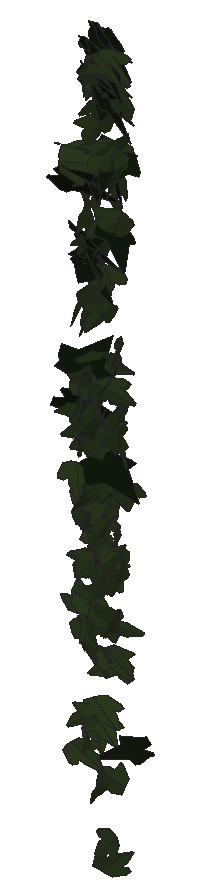
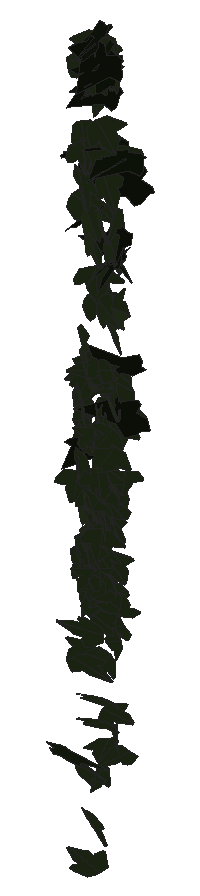
# SketchUp Ruby script. Lengths in inches.
U = 1.inch
M = Sketchup.active_model
def pt(a) = Geom::Point3d.new(a.map { |v| v * U })
def face(e, loops, mat)
  f = e.add_face(loops[0].map { |a| pt(a) })
  loops[1..].each { |l| e.add_face(l.map { |a| pt(a) }).erase! }
  f.material = f.back_material = mat if mat
  f
end
# faces: each face lists its corners as indices into pts; further lists are holes
def faces(e, pts, list, mat = nil) = list.each { |f| face(e, (f[0].is_a?(Array) ? f : [f]).map { |l| l.map { |i| pts[i] } }, mat) }
# xy, xz, yz: faces in a plane at the given z, y or x. An outline is a flat list of corners, or four numbers for a rectangle; further outlines are holes
def ring(l) = l.size == 4 ? [[l[0], l[1]], [l[2], l[1]], [l[2], l[3]], [l[0], l[3]]] : l.each_slice(2).to_a
def flat(e, list, mat, &to3) = list.each { |f| face(e, (f[0].is_a?(Array) ? f : [f]).map { |l| ring(l).map { |u, v| to3.(u, v) } }, mat) }
def xy(e, z, list, mat = nil) = flat(e, list, mat) { |x, y| [x, y, z] }
def xz(e, y, list, mat = nil) = flat(e, list, mat) { |x, z| [x, y, z] }
def yz(e, x, list, mat = nil) = flat(e, list, mat) { |y, z| [x, y, z] }
def lines(e, pts, list) = list.each { |a, b| e.add_line(pt(pts[a]), pt(pts[b])) }
# prism: a flat outline (further loops are holes) pulled along v
def prism(e, loops, v, mat = nil)
  f = face(e, loops, mat); d = Geom::Vector3d.new(v.map { |x| x * U })
  f.pushpull(f.normal.samedirection?(d) ? d.length : -d.length)
end
def box(e, o, s, mat = nil) = prism(e, [[o, [o[0] + s[0], o[1], o[2]], [o[0] + s[0], o[1] + s[1], o[2]], [o[0], o[1] + s[1], o[2]]]], [0, 0, s[2]], mat)
def at(x, y, z, deg = 0) = Geom::Transformation.translation(pt([x, y, z])) * Geom::Transformation.rotation(ORIGIN, Z_AXIS, deg.degrees)
def axes(o, x, y, z) = Geom::Transformation.new([*x, 0, *y, 0, *z, 0, *pt(o).to_a, 1])
def part(name) = M.definitions.add(name)
# library, detail: a bought-in or finely detailed component or shape, given as its bounding box
def library(name, o, s) = part(name).tap { |d| box(d.entities, o, s) }
def detail(e, o, s) = box(e.add_group.entities, o, s)
def put(e, d, t, mat = nil) = e.add_instance(d, t).tap { |i| i.material = mat if mat }
def group(e, t, mat = nil) = e.add_group.tap { |g| g.transformation = t; g.material = mat if mat }.entities
root = M.entities
M.materials.add("1026 AP 7946 SUNNY SIDE UP").color = [254, 231, 186]
M.materials.add("efeu1").color = [18, 25, 13]
M.materials.add("efeu2").color = [43, 57, 29]
c1 = part("ivyleaf_10")
p = [[0,0.5,-0.03],[-0.0625,2.02,-0.43],[-0.19,2.01,-0.46],[-0.54,1.05,-0.29],[-0.52,0.625,-0.18],[-0.83,0.76,-0.28],
  [-1.16,0.64,-0.33],[-1.15,0.33,-0.24],[-0.77,-0.39,0.02],[-0.3,-0.51,0.16],[0.04,-0.48,0.23],[-0.02,2.01,-0.4375],
  [-0.06,2.01,-0.43],[0.04,-0.49,0.23],[0.67,-0.49,0.14],[1.38,0.36,-0.2],[1.375,0.51,-0.24],[0.81,0.65,-0.19],
  [0.62,0.59,-0.15],[0.6,1.09,-0.28],[0.5,1.23,-0.31]]
faces(c1.entities,p,[[0,1,2,3,4,5,6,7,8,9,10],[11,12,0,13,14,15,16,17,18,19,20]],"efeu2")
c2 = part("ivyleaf_9")
p = [[1.54,2.16,1.25],[1.36,2.04,1.19],[-0.21,0.99,0.68],[-0.71,1.11,0.82],[-0.85,0.86,0.67],[-0.8,0.17,0.21],
  [-0.9,-0.01,0.1],[-0.67,-0.16,-0.02],[-0.08,-0.08,-0.05],[-0.03,-0.6,-0.4],[0.65,-0.88,-0.66],[0.83,-0.6,-0.49],
  [1.29,-0.42,-0.43],[1.8125,-0.07,-0.26],[1.21,0.44,0.15]]
faces(c2.entities,p,[[0,1,2,3,4,5,6,7,8,9,10,11,12,13,14]],"efeu1")
put(root,c1,axes([100.83,212.89,262.52],[0.13665,-0.19544,0.01189],[-0.00323,-0.01554,-0.22635],[0.33256,0.08016,-0.00708]),"1026 AP 7946 SUNNY SIDE UP")
put(root,c1,axes([100.85,212.84,264.03],[-0.01043,-0.23526,0.01809],[-0.0003,-0.0189,-0.24257],[0.37111,-0.00663,0.00031]),"1026 AP 7946 SUNNY SIDE UP")
put(root,c1,axes([100.76,212.64,259.7],[0.25132,0.14631,-0.00572],[0.00915,-0.01575,-0.22248],[-0.2485,0.14739,-0.01398]),"1026 AP 7946 SUNNY SIDE UP")
put(root,c2,axes([100.73,212.62,265.69],[0.37967,0.09039,0.01328],[-0.0411,0.0877,-0.23827],[-0.14905,0.20606,0.09953]),"1026 AP 7946 SUNNY SIDE UP")
put(root,c1,axes([100.84,212.66,257.16],[0.28828,0.09088,0.01076],[-0.02972,0.01592,0.2096],[0.14064,-0.18291,0.02224]),"1026 AP 7946 SUNNY SIDE UP")
put(root,c1,axes([100.77,212.8,262.84],[0.07996,-0.1274,0.21096],[0.12187,-0.19033,-0.14243],[0.36013,0.09269,0.00136]),"1026 AP 7946 SUNNY SIDE UP")
put(root,c1,axes([100.91,212.78,258.08],[-0.13223,-0.16283,0.09855],[-0.02891,-0.09816,-0.18755],[0.29628,-0.08225,0.02568]),"1026 AP 7946 SUNNY SIDE UP")
put(root,c1,axes([100.79,213.01,260.64],[-0.28985,0.02637,-0.0702],[0.10092,-0.04074,-0.18288],[-0.06588,-0.17844,0.02871]),"1026 AP 7946 SUNNY SIDE UP")
put(root,c2,axes([100.5625,212.65,260.9375],[0.09228,0.04957,-0.24052],[0.24625,0.17382,0.0795],[0.28379,-0.16695,0.00923]),"1026 AP 7946 SUNNY SIDE UP")
put(root,c1,axes([100.89,212.6,260.89],[-0.27426,-0.1545,-0.00761],[0.02677,-0.00944,-0.23935],[0.24167,-0.17429,0.01788]),"1026 AP 7946 SUNNY SIDE UP")
put(root,c1,axes([100.89,212.53,261.15],[0.09027,-0.1714,-0.14386],[-0.00129,0.14312,-0.18177],[0.34667,0.04517,0.03678]),"1026 AP 7946 SUNNY SIDE UP")
put(root,c1,axes([100.76,212.92,258.92],[0.25824,-0.10235,0.08625],[0.12248,-0.03414,-0.19922],[0.16873,0.18143,0.01261]),"1026 AP 7946 SUNNY SIDE UP")
put(root,c1,axes([100.76,213.21,264.56],[0.16686,-0.11265,0.14808],[0.14553,-0.11057,-0.16148],[0.26777,0.13029,-0.00452]),"1026 AP 7946 SUNNY SIDE UP")
put(root,c1,axes([100.63,212.77,261.42],[-0.02711,-0.01639,-0.22131],[0.29318,-0.11543,-0.00611],[-0.19419,-0.17198,0.02168]),"1026 AP 7946 SUNNY SIDE UP")
put(root,c1,axes([100.82,212.64,260.21],[-0.15831,0.14303,0.13806],[0.14235,-0.09653,0.18083],[0.29194,0.12462,-0.01331]),"1026 AP 7946 SUNNY SIDE UP")
put(root,c2,axes([100.6,212.48,265.16],[0.35763,0.03996,0.12969],[0.20161,-0.00852,-0.23633],[-0.04841,0.25971,-0.02615]),"1026 AP 7946 SUNNY SIDE UP")
put(root,c1,axes([100.91,212.77,258.98],[0.11899,-0.1979,-0.00095],[-0.00676,-0.00186,-0.21824],[0.31111,0.07565,-0.00438]),"1026 AP 7946 SUNNY SIDE UP")
put(root,c1,axes([100.86,212.71,264.49],[0.0494,-0.19948,-0.13684],[0.07459,0.13539,-0.19882],[0.36838,-0.00066,0.05861]),"1026 AP 7946 SUNNY SIDE UP")
put(root,c1,axes([100.89,213.03,257.93],[-0.27474,0.0567,-0.04591],[0.02238,-0.08242,-0.1682],[-0.11937,-0.14596,0.07414]),"1026 AP 7946 SUNNY SIDE UP")
put(root,c1,axes([100.78,213,257.7],[-0.2358,0.00664,-0.1185],[0.17399,-0.06035,-0.14231],[-0.07221,-0.1671,0.04405]),"1026 AP 7946 SUNNY SIDE UP")
put(root,c2,axes([100.87,212.69,263.85],[0.26545,-0.09188,-0.16491],[-0.22705,0.06825,-0.19747],[0.17963,0.22204,-0.0059]),"1026 AP 7946 SUNNY SIDE UP")
put(root,c1,axes([100.84,212.57,261.37],[0.04187,0.00239,0.24061],[0.00754,0.235,-0.00167],[-0.36717,0.0051,0.0274]),"1026 AP 7946 SUNNY SIDE UP")
put(root,c1,axes([100.82,212.93,257.8],[-0.17724,0.07081,-0.14009],[0.10843,-0.12422,-0.12737],[-0.22964,-0.1133,0.04799]),"1026 AP 7946 SUNNY SIDE UP")
put(root,c1,axes([100.93,212.48,259.08],[0.05187,-0.01626,0.23813],[-0.07855,0.22759,0.02516],[-0.35594,-0.0526,0.02915]),"1026 AP 7946 SUNNY SIDE UP")
put(root,c1,axes([101.02,212.6875,255.23],[-0.1167,-0.06502,0.16342],[-0.08392,-0.15062,-0.09411],[0.27025,-0.07484,0.04135]),"1026 AP 7946 SUNNY SIDE UP")
put(root,c1,axes([100.94,212.7,261.01],[0.10666,-0.21059,0.04081],[0.00753,-0.04131,-0.22802],[0.33721,0.06753,-0.00782]),"1026 AP 7946 SUNNY SIDE UP")
put(root,c1,axes([100.97,213.04,257.91],[-0.0692,-0.10126,0.14748],[-0.00023,-0.14291,-0.11343],[0.29204,-0.02411,0.03486]),"1026 AP 7946 SUNNY SIDE UP")
put(root,c1,axes([100.98,212.82,265.14],[-0.0718,-0.23668,0.02762],[-0.00268,-0.02834,-0.24846],[0.37478,-0.04555,0.00351]),"1026 AP 7946 SUNNY SIDE UP")
put(root,c1,axes([101.01,212.77,258.1],[-0.18106,-0.13037,0.1157],[-0.04366,-0.12014,-0.17256],[0.26779,-0.10773,0.05009]),"1026 AP 7946 SUNNY SIDE UP")
put(root,c1,axes([100.96,212.98,258.65],[-0.26566,-0.11815,-0.01533],[0.03451,-0.00668,-0.21162],[0.1839,-0.16942,0.01756]),"1026 AP 7946 SUNNY SIDE UP")
put(root,c1,axes([100.98,212.87,262.85],[0.00658,-0.2045,0.11564],[0.0091,-0.1133,-0.21135],[0.36757,0.00646,0.00316]),"1026 AP 7946 SUNNY SIDE UP")
put(root,c1,axes([100.78,212.62,254.52],[0.15606,0.11813,0.14604],[0.16222,0.09701,-0.15788],[-0.23959,0.14264,-0.01178]),"1026 AP 7946 SUNNY SIDE UP")
put(root,c1,axes([101.07,212.61,261.21],[-0.12313,0.15192,-0.16471],[-0.09578,0.14912,0.17663],[0.33434,0.09867,-0.01006]),"1026 AP 7946 SUNNY SIDE UP")
put(root,c1,axes([100.98,212.77,258.98],[-0.03758,-0.19625,0.06368],[0.01359,-0.06425,-0.20341],[0.32377,-0.02008,0.01593]),"1026 AP 7946 SUNNY SIDE UP")
put(root,c2,axes([100.85,212.625,261.58],[-0.18274,-0.00375,0.22652],[0.33447,0.06129,0.11724],[-0.08789,0.24105,-0.02479]),"1026 AP 7946 SUNNY SIDE UP")
put(root,c1,axes([100.9,212.83,260.15],[-0.31442,-0.05777,-0.07811],[0.12679,-0.00996,-0.21224],[0.07917,-0.2135,0.02969]),"1026 AP 7946 SUNNY SIDE UP")
put(root,c1,axes([100.95,212.68,267.12],[-0.27533,0.18064,-0.02232],[0.00585,-0.02792,-0.25877],[-0.28622,-0.17434,0.01618]),"1026 AP 7946 SUNNY SIDE UP")
put(root,c1,axes([101.03,212.9,266.17],[-0.1391,-0.21122,0.09816],[-0.01901,-0.09892,-0.23509],[0.36464,-0.08573,0.02519]),"1026 AP 7946 SUNNY SIDE UP")
put(root,c1,axes([100.9,212.94,254.83],[0.12092,0.19268,0.01725],[0.01968,0.01185,-0.21353],[-0.30334,0.07758,-0.00698]),"1026 AP 7946 SUNNY SIDE UP")
put(root,c1,axes([100.98,212.75,258.96],[-0.01835,-0.18616,-0.09728],[0.02667,0.09236,-0.19134],[0.32638,-0.01801,0.01017]),"1026 AP 7946 SUNNY SIDE UP")
put(root,c1,axes([100.98,212.5625,261.33],[0.01684,-0.02935,0.23079],[-0.0714,0.21959,0.03313],[-0.34828,-0.04644,0.00437]),"1026 AP 7946 SUNNY SIDE UP")
put(root,c1,axes([101.01,212.69,259.7],[0.10256,-0.21321,0.01528],[0.00009,-0.01676,-0.22974],[0.3362,0.06504,-0.0046]),"1026 AP 7946 SUNNY SIDE UP")
put(root,c2,axes([101.19,212.7,263.99],[-0.21293,0.19926,0.01856],[-0.02391,0.01007,-0.24803],[-0.31353,-0.13609,0.00632]),"1026 AP 7946 SUNNY SIDE UP")
put(root,c1,axes([100.78,212.81,259.21],[0.23154,0.04263,0.14785],[0.2289,0.02869,-0.15227],[-0.0858,0.19158,-0.00723]),"1026 AP 7946 SUNNY SIDE UP")
put(root,c1,axes([101.05,212.87,261.78],[-0.14826,-0.1957,0.06223],[-0.01221,-0.06425,-0.22321],[0.32234,-0.09245,0.02017]),"1026 AP 7946 SUNNY SIDE UP")
put(root,c1,axes([101,212.6,260.53],[-0.29341,-0.13473,-0.04142],[0.07203,0.00358,-0.23584],[0.20867,-0.19069,0.02317]),"1026 AP 7946 SUNNY SIDE UP")
put(root,c2,axes([100.9,212.89,265.42],[-0.01736,-0.24334,0.02718],[-0.00489,-0.02765,-0.2511],[0.38509,-0.01132,-0.00196]),"1026 AP 7946 SUNNY SIDE UP")
put(root,c1,axes([100.85,213.16,259.39],[0.24045,-0.01826,0.11366],[0.17273,-0.03608,-0.15215],[0.06126,0.17345,-0.01713]),"1026 AP 7946 SUNNY SIDE UP")
put(root,c1,axes([100.99,212.95,259.18],[0.32968,-0.01453,-0.01541],[-0.02335,0.0008,-0.21651],[0.02288,0.21019,0.00099]),"1026 AP 7946 SUNNY SIDE UP")
put(root,c1,axes([100.89,212.67,256.6],[-0.13309,0.08738,-0.16907],[0.13988,-0.13992,-0.12446],[-0.2575,-0.12117,0.01977]),"1026 AP 7946 SUNNY SIDE UP")
put(root,c1,axes([101.07,212.93,259.71],[-0.26038,-0.13156,0.02314],[-0.00356,-0.0342,-0.21653],[0.21003,-0.16368,0.02502]),"1026 AP 7946 SUNNY SIDE UP")
put(root,c1,axes([101.05,212.62,260.69],[-0.01078,-0.20799,-0.11388],[0.01391,0.1091,-0.2137],[0.36924,-0.01018,0.00472]),"1026 AP 7946 SUNNY SIDE UP")
put(root,c2,axes([100.74,212.75,263.98],[0.23493,-0.11998,0.14136],[0.15237,-0.09988,-0.19696],[0.26402,0.1644,-0.01212]),"1026 AP 7946 SUNNY SIDE UP")
put(root,c1,axes([100.76,212.47,265.52],[0.07599,-0.06377,-0.26869],[0.37301,0.13355,0.01244],[0.19657,-0.22877,0.08026]),"1026 AP 7946 SUNNY SIDE UP")
put(root,c1,axes([100.98,212.85,256.32],[-0.27454,0.09393,-0.072],[0.08068,-0.05246,-0.20344],[-0.16603,-0.18081,0.02019]),"1026 AP 7946 SUNNY SIDE UP")
put(root,c2,axes([100.93,212.93,267.54],[0.38638,0.04371,-0.06044],[-0.08599,-0.02816,-0.25664],[-0.07689,0.25112,-0.01672]),"1026 AP 7946 SUNNY SIDE UP")
put(root,c1,axes([101.08,212.88,267.12],[-0.09157,-0.21523,0.12411],[0.00942,-0.12622,-0.22775],[0.38867,-0.04765,0.03476]),"1026 AP 7946 SUNNY SIDE UP")
put(root,c1,axes([100.88,212.69,254.75],[-0.02542,0.0368,0.20998],[0.24142,-0.13478,0.03687],[0.21811,0.15348,-0.01633]),"1026 AP 7946 SUNNY SIDE UP")
put(root,c1,axes([101.08,212.75,267.22],[0.01266,-0.25141,0.06095],[0.00294,-0.06056,-0.25949],[0.40663,0.00827,-0.00002]),"1026 AP 7946 SUNNY SIDE UP")
put(root,c1,axes([100.85,212.61,256.86],[0.18095,-0.02457,0.15651],[0.24549,-0.0241,-0.11731],[0.05771,0.17958,0.00827]),"1026 AP 7946 SUNNY SIDE UP")
put(root,c1,axes([101.01,212.93,258.38],[0.32581,-0.06354,0.01471],[0.01261,-0.02357,-0.22244],[0.10175,0.20638,-0.01954]),"1026 AP 7946 SUNNY SIDE UP")
put(root,c1,axes([100.94,212.86,259.42],[-0.26232,0.03497,-0.12602],[0.15923,-0.08953,-0.16095],[-0.13566,-0.1727,0.05475]),"1026 AP 7946 SUNNY SIDE UP")
put(root,c1,axes([101.11,212.91,259.32],[-0.10497,-0.20356,0.00748],[0.00258,-0.0094,-0.2207],[0.32034,-0.06663,0.00423]),"1026 AP 7946 SUNNY SIDE UP")
put(root,c1,axes([100.87,212.8125,258.9375],[0.16736,0.10312,0.16387],[0.19404,0.09991,-0.15176],[-0.22526,0.16268,-0.00898]),"1026 AP 7946 SUNNY SIDE UP")
put(root,c1,axes([101.16,212.76,256.92],[-0.14689,-0.11703,0.14941],[-0.05437,-0.14925,-0.14722],[0.28878,-0.08763,0.04828]),"1026 AP 7946 SUNNY SIDE UP")
put(root,c2,axes([100.79,212.95,267.28],[0.26797,-0.15915,0.10566],[0.11374,-0.07411,-0.24061],[0.27596,0.18509,-0.00343]),"1026 AP 7946 SUNNY SIDE UP")
put(root,c1,axes([100.95,212.56,257.42],[0.0752,0.11898,0.18136],[0.1145,0.15961,-0.13108],[-0.31294,0.08699,-0.00438]),"1026 AP 7946 SUNNY SIDE UP")
put(root,c2,axes([100.94,212.65,263.64],[0.14502,-0.20446,-0.10143],[-0.05136,0.09195,-0.2304],[0.35231,0.09756,0.00816]),"1026 AP 7946 SUNNY SIDE UP")
put(root,c1,axes([101.13,212.92,259.37],[0.17752,-0.15811,-0.08935],[-0.04252,0.08527,-0.19796],[0.27967,0.11332,0.02662]),"1026 AP 7946 SUNNY SIDE UP")
put(root,c1,axes([101.27,212.73,257.03],[-0.20132,-0.0714,-0.15896],[-0.22844,-0.05342,0.14974],[-0.13776,0.19293,-0.016]),"1026 AP 7946 SUNNY SIDE UP")
put(root,c1,axes([101.13,212.92,258.32],[-0.01379,-0.18974,0.07129],[0.01625,-0.07067,-0.19565],[0.31774,-0.00462,0.0131]),"1026 AP 7946 SUNNY SIDE UP")
put(root,c1,axes([101.15,212.89,263.41],[-0.28891,-0.14894,0.02382],[0.04546,-0.07183,-0.23198],[0.23281,-0.1708,0.07485]),"1026 AP 7946 SUNNY SIDE UP")
put(root,c1,axes([101.02,212.8,267.14],[0.12687,0.22667,0.08587],[0.06934,0.07121,-0.24685],[-0.37267,0.09041,-0.0167]),"1026 AP 7946 SUNNY SIDE UP")
put(root,c1,axes([101.17,212.67,267.5],[-0.0194,-0.25348,-0.02101],[0.01779,0.01841,-0.26112],[0.39929,-0.01314,0.01061]),"1026 AP 7946 SUNNY SIDE UP")
put(root,c1,axes([101.2,212.8,257.6],[-0.09268,-0.18925,0.07614],[-0.0166,-0.07511,-0.2043],[0.31965,-0.05877,0.01147]),"1026 AP 7946 SUNNY SIDE UP")
put(root,c1,axes([101.17,212.93,259.29],[-0.1828,-0.17721,-0.01701],[0.04216,0.00086,-0.21717],[0.27652,-0.11728,0.02186]),"1026 AP 7946 SUNNY SIDE UP")
put(root,c1,axes([101.18,212.8,258.6875],[0.00379,-0.1708,0.12756],[0.00432,-0.12476,-0.1767],[0.33258,0.00357,0.00084]),"1026 AP 7946 SUNNY SIDE UP")
put(root,c2,axes([101.07,212.94,267.04],[-0.06185,-0.23789,0.07333],[-0.01621,-0.07181,-0.24881],[0.39072,-0.04064,0.00129]),"1026 AP 7946 SUNNY SIDE UP")
put(root,c1,axes([101.01,213,260.51],[0.21077,0.10361,0.09917],[0.13654,0.04552,-0.1718],[-0.19055,0.14723,-0.0134]),"1026 AP 7946 SUNNY SIDE UP")
put(root,c1,axes([101.21,212.96,264.47],[0.00723,-0.23714,0.02324],[0.00007,-0.02391,-0.24449],[0.37477,0.00458,-0.0004]),"1026 AP 7946 SUNNY SIDE UP")
put(root,c1,axes([101.19,212.82,257.875],[-0.04149,-0.1907,0.07084],[0.02781,-0.07232,-0.19696],[0.31812,-0.01855,0.02645]),"1026 AP 7946 SUNNY SIDE UP")
put(root,c1,axes([101.27,212.76,262.8],[-0.09854,-0.17164,0.14094],[-0.04642,-0.13542,-0.1884],[0.34296,-0.06765,0.015]),"1026 AP 7946 SUNNY SIDE UP")
put(root,c1,axes([101.23,212.96,259.27],[0.05229,-0.20722,0.02212],[-0.00798,-0.02374,-0.21616],[0.32767,0.03249,-0.0088]),"1026 AP 7946 SUNNY SIDE UP")
put(root,c1,axes([101.04,212.97,257.87],[0.22756,0.12146,0.10955],[0.14338,0.05523,-0.19377],[-0.20861,0.17046,-0.01367]),"1026 AP 7946 SUNNY SIDE UP")
put(root,c1,axes([101.25,212.58,260.78],[0.0102,-0.23889,-0.05888],[-0.01069,0.05562,-0.24581],[0.38559,0.00786,-0.00526]),"1026 AP 7946 SUNNY SIDE UP")
put(root,c1,axes([101.28,212.99,265.72],[-0.28825,-0.14405,0.07281],[-0.01515,-0.09838,-0.23023],[0.25241,-0.17041,0.06933]),"1026 AP 7946 SUNNY SIDE UP")
put(root,c1,axes([101.23,212.72,260.64],[0.19498,-0.15588,-0.10766],[-0.00601,0.12215,-0.19332],[0.29425,0.10578,0.06738]),"1026 AP 7946 SUNNY SIDE UP")
put(root,c1,axes([101.27,212.74,259.09],[-0.17753,-0.15334,0.08953],[0.00155,-0.10472,-0.18775],[0.27782,-0.0974,0.05826]),"1026 AP 7946 SUNNY SIDE UP")
put(root,c2,axes([101.02,212.72,266.89],[0.39375,-0.03489,0.00603],[0.00431,-0.024,-0.25949],[0.05551,0.24934,-0.02263]),"1026 AP 7946 SUNNY SIDE UP")
put(root,c1,axes([101.01,212.89,261.66],[0.08571,-0.00758,0.2042],[0.23393,0.13812,-0.03123],[-0.22448,0.14104,0.04542]),"1026 AP 7946 SUNNY SIDE UP")
put(root,c2,axes([101.07,212.97,267.77],[0.08851,-0.24664,0.03802],[0.0027,-0.03889,-0.26075],[0.39246,0.05589,-0.00678]),"1026 AP 7946 SUNNY SIDE UP")
put(root,c2,axes([101.16,212.98,266.84],[-0.0975,-0.21625,0.11179],[-0.00298,-0.11284,-0.23083],[0.38131,-0.05618,0.02678]),"1026 AP 7946 SUNNY SIDE UP")
put(root,c1,axes([101.27,212.84,264.01],[0.01208,-0.2398,0.0051],[0.00123,-0.00629,-0.2472],[0.37719,0.0077,0.00064]),"1026 AP 7946 SUNNY SIDE UP")
put(root,c1,axes([101.25,212.83,257.91],[0.11248,-0.19027,0.02663],[0.00494,-0.02757,-0.20946],[0.30212,0.07129,-0.00649]),"1026 AP 7946 SUNNY SIDE UP")
put(root,c1,axes([101.38,212.96,256.17],[0.24219,0.00971,-0.15782],[-0.23465,-0.04169,-0.15748],[-0.0569,0.21324,-0.02231]),"1026 AP 7946 SUNNY SIDE UP")
put(root,c1,axes([101.11,212.82,255.0625],[-0.23928,-0.10344,-0.07563],[0.21119,-0.11299,-0.09194],[0.00814,-0.1091,0.16239]),"1026 AP 7946 SUNNY SIDE UP")
put(root,c1,axes([101.08,212.72,263.24],[0.16975,-0.08534,0.20073],[0.24216,-0.12014,-0.14247],[0.23172,0.18808,0.00185]),"1026 AP 7946 SUNNY SIDE UP")
put(root,c1,axes([101.27,212.54,254.02],[-0.01521,-0.11172,-0.18951],[0.04295,0.18138,-0.1143],[0.33482,-0.02834,0.00605]),"1026 AP 7946 SUNNY SIDE UP")
put(root,c2,axes([101.0625,212.89,267.42],[0.15846,-0.24723,0.06203],[0.0117,-0.06337,-0.27488],[0.40046,0.09968,-0.01651]),"1026 AP 7946 SUNNY SIDE UP")
put(root,c1,axes([101.28,212.6,266.77],[-0.11267,-0.23637,-0.08029],[0.05373,0.06959,-0.25374],[0.38698,-0.07848,0.01186]),"1026 AP 7946 SUNNY SIDE UP")
put(root,c1,axes([101.4,212.71,265.76],[-0.27381,-0.12325,0.13131],[-0.10224,-0.12281,-0.21342],[0.26022,-0.17794,0.05431]),"1026 AP 7946 SUNNY SIDE UP")
put(root,c1,axes([101.35,212.91,258.24],[-0.19332,-0.1416,0.08758],[-0.03934,-0.08978,-0.19005],[0.25736,-0.12008,0.03674]),"1026 AP 7946 SUNNY SIDE UP")
put(root,c1,axes([101.27,212.73,263.13],[-0.03467,0.16099,0.18281],[0.06854,-0.1716,0.16582],[0.36938,0.04695,-0.01361]),"1026 AP 7946 SUNNY SIDE UP")
put(root,c1,axes([101.31,212.97,259.03],[0.02439,-0.20774,0.0163],[-0.0001,-0.01705,-0.2147],[0.32774,0.01545,-0.00128]),"1026 AP 7946 SUNNY SIDE UP")
put(root,c2,axes([101.07,212.96,267.77],[0.20318,-0.21492,0.05184],[0.01798,-0.05312,-0.25805],[0.34706,0.12858,-0.01698]),"1026 AP 7946 SUNNY SIDE UP")
put(root,c1,axes([101.15,212.73,255.43],[-0.23515,-0.11263,-0.10114],[0.2467,-0.11911,-0.07899],[-0.02482,-0.11684,0.17316]),"1026 AP 7946 SUNNY SIDE UP")
put(root,c1,axes([101.35,212.88,260.58],[0.20609,-0.16383,-0.07148],[-0.03481,0.06934,-0.21423],[0.27701,0.1306,0.02625]),"1026 AP 7946 SUNNY SIDE UP")
put(root,c1,axes([101.54,212.78,254.07],[0.05339,0.0519,0.20112],[-0.31592,0.02634,0.02899],[-0.0283,-0.19611,0.05587]),"1026 AP 7946 SUNNY SIDE UP")
put(root,c1,axes([101.36,212.93,258.48],[0.10379,-0.1879,-0.04477],[-0.02138,0.04016,-0.20493],[0.30212,0.06739,0.00088]),"1026 AP 7946 SUNNY SIDE UP")
put(root,c1,axes([101.23,212.85,252.36],[-0.16048,-0.12428,0.13801],[0.11598,0.11325,0.16592],[-0.26377,0.12541,-0.01101]),"1026 AP 7946 SUNNY SIDE UP")
put(root,c1,axes([101.35,212.98,265.18],[0.28764,-0.14528,-0.06244],[-0.02176,0.0765,-0.2347],[0.24606,0.17659,0.05223]),"1026 AP 7946 SUNNY SIDE UP")
put(root,c1,axes([101.35,212.93,265.7],[0.12426,-0.22948,-0.05179],[0.02808,0.0574,-0.24711],[0.36789,0.07313,0.03635]),"1026 AP 7946 SUNNY SIDE UP")
put(root,c1,axes([101.38,212.71,261.4375],[0.05953,-0.22345,0.06912],[0.00143,-0.06911,-0.23364],[0.36742,0.03647,-0.01029]),"1026 AP 7946 SUNNY SIDE UP")
put(root,c2,axes([101.36,212.98,265.64],[-0.22817,-0.19519,0.03022],[0.01301,-0.04375,-0.24857],[0.31036,-0.14167,0.03264]),"1026 AP 7946 SUNNY SIDE UP")
put(root,c1,axes([101.39,212.73,258.37],[-0.0076,-0.20687,-0.01948],[0.00628,0.01764,-0.21304],[0.32642,-0.00516,0.00364]),"1026 AP 7946 SUNNY SIDE UP")
put(root,c1,axes([101.12,212.98,256.81],[-0.01323,-0.01518,-0.22252],[0.33979,-0.01275,-0.00782],[-0.01915,-0.2157,0.01485]),"1026 AP 7946 SUNNY SIDE UP")
put(root,c1,axes([101.55,212.75,264.5625],[-0.14808,-0.12489,0.20813],[-0.15561,-0.17777,-0.16121],[0.34054,-0.13553,0.01684]),"1026 AP 7946 SUNNY SIDE UP")
put(root,c1,axes([101.41,212.87,261.76],[0.11969,-0.21368,-0.01358],[-0.00585,0.01138,-0.23362],[0.33647,0.07621,0.00077]),"1026 AP 7946 SUNNY SIDE UP")
put(root,c1,axes([101.43,212.8125,257.89],[-0.12381,-0.19542,0.00813],[0.0055,-0.0111,-0.21698],[0.30755,-0.07847,0.00715]),"1026 AP 7946 SUNNY SIDE UP")
put(root,c1,axes([101.55,212.83,261.14],[-0.10579,0.14807,0.15494],[-0.2118,0.09034,-0.15404],[-0.25426,-0.13686,0.06385]),"1026 AP 7946 SUNNY SIDE UP")
put(root,c1,axes([101.46,212.82,265.94],[-0.08101,-0.24226,-0.02471],[0.00807,0.02203,-0.25503],[0.3825,-0.05177,0.00015]),"1026 AP 7946 SUNNY SIDE UP")
put(root,c1,axes([101.4,212.8,261.34],[-0.13453,-0.18374,-0.10726],[0.08539,0.08825,-0.208],[0.32008,-0.10077,0.01041]),"1026 AP 7946 SUNNY SIDE UP")
put(root,c1,axes([101.46,212.79,258.3],[-0.04107,-0.20941,0.02672],[-0.00015,-0.02733,-0.21753],[0.33202,-0.02591,0.00321]),"1026 AP 7946 SUNNY SIDE UP")
put(root,c1,axes([101.52,212.57,253.07],[0.22398,-0.13787,-0.08862],[-0.11515,0.04649,-0.20328],[0.22738,0.15936,-0.01565]),"1026 AP 7946 SUNNY SIDE UP")
put(root,c1,axes([101.5,212.76,264.71],[0.1668,-0.17323,-0.14015],[-0.06338,0.13209,-0.20637],[0.33953,0.10976,0.03033]),"1026 AP 7946 SUNNY SIDE UP")
put(root,c1,axes([101.47,212.84,262.12],[0.1305,-0.214,-0.03164],[-0.01203,0.02867,-0.23627],[0.33946,0.08329,0.00379]),"1026 AP 7946 SUNNY SIDE UP")
put(root,c2,axes([101.53,212.68,265.39],[0.1552,-0.05656,-0.23427],[-0.33346,0.0826,-0.11567],[0.15561,0.23343,-0.01422]),"1026 AP 7946 SUNNY SIDE UP")
put(root,c2,axes([101.66,213.21,254.54],[-0.34509,0.06338,-0.00686],[-0.04915,-0.11321,-0.19231],[-0.09649,-0.169,0.1225]),"1026 AP 7946 SUNNY SIDE UP")
put(root,c1,axes([101.34,212.6,267.56],[-0.24128,-0.16068,-0.13635],[0.23749,0.02571,-0.21389],[0.22393,-0.2004,0.07993]),"1026 AP 7946 SUNNY SIDE UP")
put(root,c1,axes([101.46,212.9,259.9],[0.24605,-0.14439,-0.0354],[0.02636,0.0657,-0.2104],[0.23159,0.14592,0.06156]),"1026 AP 7946 SUNNY SIDE UP")
put(root,c1,axes([101.39,212.89,260.39],[-0.18327,0.13072,-0.13624],[0.10723,-0.11609,-0.1798],[-0.27291,-0.1334,0.02085]),"1026 AP 7946 SUNNY SIDE UP")
put(root,c2,axes([101.3,212.65,266.86],[0.20329,-0.21691,0.00482],[-0.0086,-0.01014,-0.26],[0.34108,0.12902,-0.00943]),"1026 AP 7946 SUNNY SIDE UP")
put(root,c1,axes([101.31,212.82,256.35],[0.21236,0.07813,0.14104],[0.19523,0.05741,-0.16011],[-0.15173,0.18321,-0.00861]),"1026 AP 7946 SUNNY SIDE UP")
put(root,c1,axes([101.52,212.78,265.45],[0.10141,-0.23123,0.0577],[0.01262,-0.05724,-0.24752],[0.37438,0.06456,-0.00728]),"1026 AP 7946 SUNNY SIDE UP")
put(root,c2,axes([101.39,212.83,264.35],[0.022,-0.2412,0.0079],[-0.00396,-0.0092,-0.24894],[0.37951,0.01389,-0.00305]),"1026 AP 7946 SUNNY SIDE UP")
put(root,c1,axes([101.52,212.91,259.51],[-0.29728,-0.0968,-0.01864],[0.04637,-0.0195,-0.21663],[0.14758,-0.18887,0.03051]),"1026 AP 7946 SUNNY SIDE UP")
put(root,c1,axes([101.47,212.5,258.29],[0.03355,0.04692,-0.21629],[0.10265,0.1999,0.05396],[0.32275,-0.06845,0.00532]),"1026 AP 7946 SUNNY SIDE UP")
put(root,c2,axes([101.37,212.59,260.06],[-0.02951,-0.14203,-0.21328],[0.07525,0.20095,-0.14589],[0.38647,-0.04997,0.01212]),"1026 AP 7946 SUNNY SIDE UP")
put(root,c1,axes([101.54,212.83,258.06],[0.10061,-0.17988,-0.07819],[0.00164,0.07913,-0.19445],[0.30637,0.05865,0.02672]),"1026 AP 7946 SUNNY SIDE UP")
put(root,c1,axes([101.57,212.74,260.99],[-0.02697,-0.21769,0.02587],[-0.00112,-0.02637,-0.22511],[0.34479,-0.01711,0.0013]),"1026 AP 7946 SUNNY SIDE UP")
put(root,c1,axes([101.38,212.57,261.48],[-0.18303,-0.08965,-0.18228],[0.25068,0.0788,-0.14915],[0.18438,-0.19613,0.02182]),"1026 AP 7946 SUNNY SIDE UP")
put(root,c1,axes([101.76,212.6,266.97],[-0.24688,0.12382,0.16409],[-0.27647,0.01334,-0.18999],[-0.15379,-0.22276,0.07812]),"1026 AP 7946 SUNNY SIDE UP")
put(root,c1,axes([101.6,212.63,260.65],[-0.05244,-0.21325,-0.05989],[0.02721,0.05487,-0.22187],[0.34599,-0.03664,0.00837]),"1026 AP 7946 SUNNY SIDE UP")
put(root,c1,axes([101.61,212.55,257.21],[-0.00414,-0.17562,-0.12562],[0.01578,0.12072,-0.1801],[0.33492,-0.00786,0.00693]),"1026 AP 7946 SUNNY SIDE UP")
